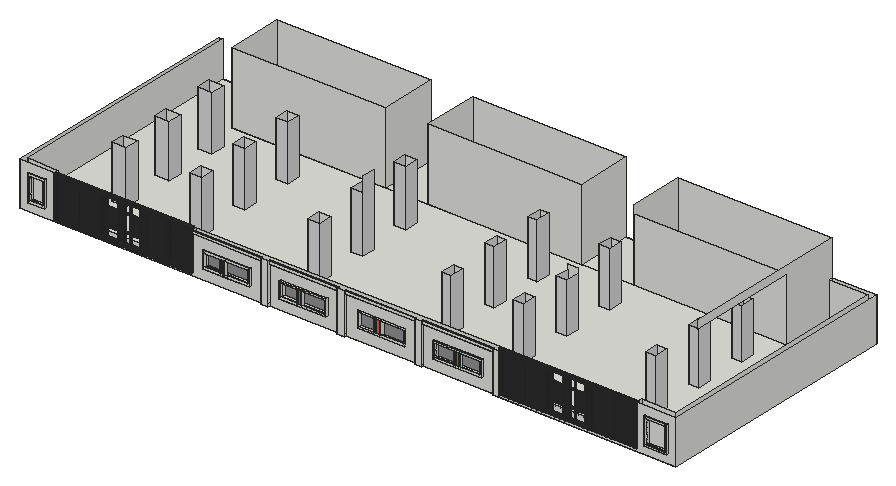
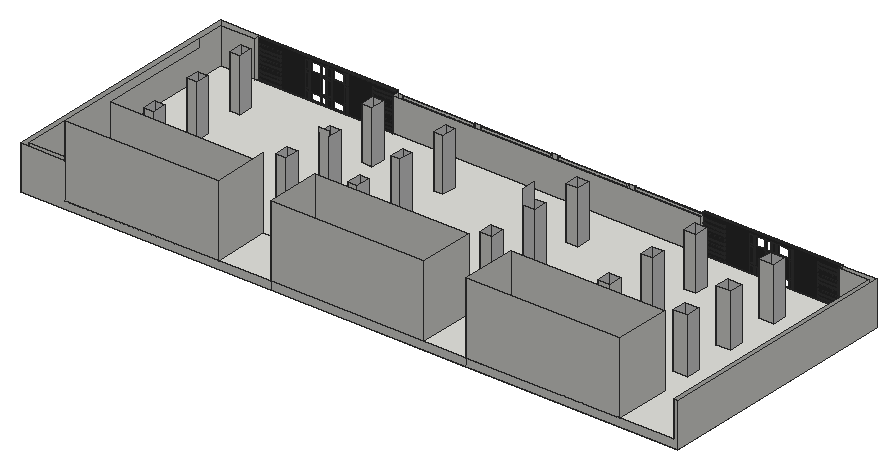
# SketchUp Ruby script. Lengths in inches.
U = 1.inch
M = Sketchup.active_model
def pt(a) = Geom::Point3d.new(a.map { |v| v * U })
def face(e, loops, mat)
  f = e.add_face(loops[0].map { |a| pt(a) })
  loops[1..].each { |l| e.add_face(l.map { |a| pt(a) }).erase! }
  f.material = f.back_material = mat if mat
  f
end
# faces: each face lists its corners as indices into pts; further lists are holes
def faces(e, pts, list, mat = nil) = list.each { |f| face(e, (f[0].is_a?(Array) ? f : [f]).map { |l| l.map { |i| pts[i] } }, mat) }
# xy, xz, yz: faces in a plane at the given z, y or x. An outline is a flat list of corners, or four numbers for a rectangle; further outlines are holes
def ring(l) = l.size == 4 ? [[l[0], l[1]], [l[2], l[1]], [l[2], l[3]], [l[0], l[3]]] : l.each_slice(2).to_a
def flat(e, list, mat, &to3) = list.each { |f| face(e, (f[0].is_a?(Array) ? f : [f]).map { |l| ring(l).map { |u, v| to3.(u, v) } }, mat) }
def xy(e, z, list, mat = nil) = flat(e, list, mat) { |x, y| [x, y, z] }
def xz(e, y, list, mat = nil) = flat(e, list, mat) { |x, z| [x, y, z] }
def yz(e, x, list, mat = nil) = flat(e, list, mat) { |y, z| [x, y, z] }
def lines(e, pts, list) = list.each { |a, b| e.add_line(pt(pts[a]), pt(pts[b])) }
# prism: a flat outline (further loops are holes) pulled along v
def prism(e, loops, v, mat = nil)
  f = face(e, loops, mat); d = Geom::Vector3d.new(v.map { |x| x * U })
  f.pushpull(f.normal.samedirection?(d) ? d.length : -d.length)
end
def box(e, o, s, mat = nil) = prism(e, [[o, [o[0] + s[0], o[1], o[2]], [o[0] + s[0], o[1] + s[1], o[2]], [o[0], o[1] + s[1], o[2]]]], [0, 0, s[2]], mat)
def at(x, y, z, deg = 0) = Geom::Transformation.translation(pt([x, y, z])) * Geom::Transformation.rotation(ORIGIN, Z_AXIS, deg.degrees)
def axes(o, x, y, z) = Geom::Transformation.new([*x, 0, *y, 0, *z, 0, *pt(o).to_a, 1])
def part(name) = M.definitions.add(name)
# library, detail: a bought-in or finely detailed component or shape, given as its bounding box
def library(name, o, s) = part(name).tap { |d| box(d.entities, o, s) }
def detail(e, o, s) = box(e.add_group.entities, o, s)
def put(e, d, t, mat = nil) = e.add_instance(d, t).tap { |i| i.material = mat if mat }
def group(e, t, mat = nil) = e.add_group.tap { |g| g.transformation = t; g.material = mat if mat }.entities
root = M.entities
M.materials.add("Generic").color = [145, 145, 145]
M.materials.add("Generic\#2").color = [229, 87, 87]
M.materials.add("Generic\#3").color = [216, 216, 216]
M.materials.add("[Color M08]").color = [45, 45, 45]
c1 = part("Group\#13")
xy(c1.entities,0,[[0,0,323.37,7]],"[Color M08]")
xy(c1.entities,5.37,[[5.37,0,53,7],[58.37,0,106,4],[111.37,0,159,0,159,7,150.06,7,150.06,4,148.06,4,148.06,7,121.81,7,121.81,4,119.81,4,119.81,7,111.37,7],[164.37,0,212,0,212,7,201.24,7,201.24,4,199.24,4,199.24,7,176.81,7,176.81,4,174.81,4,174.81,7,164.37,7],[217.37,0,265,4],
  [270.37,0,318,4]],"[Color M08]")
xy(c1.entities,8.44,[[5.37,4,53,7]])
xy(c1.entities,8.57,[[270.37,4,318,7]],"[Color M08]")
xy(c1.entities,12.19,[[270.37,4,318,7]],"[Color M08]")
xy(c1.entities,13.07,[[5.37,4,53,7]],"[Color M08]")
xy(c1.entities,16.32,[[5.37,4,53,7]],"[Color M08]")
xy(c1.entities,17.82,[[270.37,4,318,7]],"[Color M08]")
xy(c1.entities,20.94,[[5.37,4,53,7]],"[Color M08]")
xy(c1.entities,21.44,[[270.37,4,318,7]],"[Color M08]")
xy(c1.entities,24.19,[[5.37,4,53,7]],"[Color M08]")
xy(c1.entities,26.69,[[111.37,4,119.81,7],[121.81,4,148.06,7],[150.06,4,159,7],[164.37,4,174.81,7],[176.81,4,199.24,7],
  [201.24,4,212,7]],"[Color M08]")
xy(c1.entities,27.07,[[270.37,4,318,7]],"[Color M08]")
xy(c1.entities,28.82,[[5.37,4,53,7]],"[Color M08]")
xy(c1.entities,29.69,[[111.37,4,119.81,7],[150.06,4,159,7],[164.37,4,174.81,7],[201.24,4,212,7]],"[Color M08]")
xy(c1.entities,30.69,[[270.37,4,318,7]],"[Color M08]")
xy(c1.entities,32.07,[[5.37,4,53,7]],"[Color M08]")
xy(c1.entities,36.32,[[270.37,4,318,7]],"[Color M08]")
xy(c1.entities,36.69,[[5.37,4,53,7]],"[Color M08]")
xy(c1.entities,39.94,[[5.37,4,53,7],[270.37,4,318,7]],"[Color M08]")
xy(c1.entities,44.57,[[5.37,4,53,7]],"[Color M08]")
xy(c1.entities,45.57,[[270.37,4,318,7]],"[Color M08]")
xy(c1.entities,47.82,[[5.37,4,53,7]],"[Color M08]")
xy(c1.entities,49.19,[[270.37,4,318,7]],"[Color M08]")
xy(c1.entities,52.44,[[5.37,4,53,7]],"[Color M08]")
xy(c1.entities,54.82,[[270.37,4,318,7]],"[Color M08]")
xy(c1.entities,55.69,[[5.37,4,53,7]],"[Color M08]")
xy(c1.entities,58.44,[[270.37,4,318,7]],"[Color M08]")
xy(c1.entities,60.32,[[5.37,4,53,7]],"[Color M08]")
xy(c1.entities,63.57,[[5.37,4,53,7]],"[Color M08]")
xy(c1.entities,64.07,[[270.37,4,318,7]],"[Color M08]")
xy(c1.entities,66.38,[[111.37,4,119.81,7],[150.06,4,159,7],[164.37,4,174.81,7],[201.24,4,212,7]],"[Color M08]")
xy(c1.entities,67.69,[[270.37,4,318,7]],"[Color M08]")
xy(c1.entities,68.19,[[5.37,4,53,7]],"[Color M08]")
xy(c1.entities,69.38,[[111.37,4,119.81,7],[121.81,4,148.06,7],[150.06,4,159,7],[164.37,4,174.81,7],[176.81,4,199.24,7],
  [201.24,4,212,7]],"[Color M08]")
xy(c1.entities,71.44,[[5.37,4,53,7]],"[Color M08]")
xy(c1.entities,73.32,[[270.37,4,318,7]],"[Color M08]")
xy(c1.entities,76.07,[[5.37,4,53,7]],"[Color M08]")
xy(c1.entities,76.94,[[270.37,4,318,7]],"[Color M08]")
xy(c1.entities,79.32,[[5.37,4,53,7]],"[Color M08]")
xy(c1.entities,82.57,[[270.37,4,318,7]],"[Color M08]")
xy(c1.entities,83.94,[[5.37,4,53,7]],"[Color M08]")
xy(c1.entities,86.19,[[270.37,4,318,7]],"[Color M08]")
xy(c1.entities,87.19,[[5.37,4,53,7]],"[Color M08]")
xy(c1.entities,91.82,[[5.37,0,53,4],[58.37,0,106,4],[111.37,0,111.37,7,119.81,7,119.81,4,121.81,4,121.81,7,148.06,7,148.06,4,150.06,4,150.06,7,159,7,159,0],[164.37,0,164.37,7,174.81,7,174.81,4,176.81,4,176.81,7,199.24,7,199.24,4,201.24,4,201.24,7,212,7,212,0],[217.37,0,265,4],
  [270.37,0,318,4]],"[Color M08]")
xy(c1.entities,97.1875,[[0,0,323.37,7]],"[Color M08]")
xz(c1.entities,0,[[[0,0,323.37,0,323.37,97.1875,0,97.1875,0,5.37,5.37,5.37,5.37,91.82,53,91.82,53,5.37,58.37,5.37,58.37,91.82,106,91.82,106,5.37,111.37,5.37,111.37,91.82,212,91.82,212,5.37,0,5.37],[270.37,5.37,318,91.82],[217.37,5.37,265,91.82]],[159,5.37,164.37,91.82]],"[Color M08]")
xz(c1.entities,4,[[5.37,0.57,53,5.19],[270.37,2.94,318,5.37]])
xz(c1.entities,4,[[58.37,5.37,106,91.82],[119.81,5.37,121.81,5.37,121.81,26.69,148.06,26.69,148.06,5.37,150.06,5.37,150.06,26.69,159,26.69,159,29.69,150.06,29.69,150.06,66.38,159,66.38,159,69.38,150.06,69.38,150.06,91.82,148.06,91.82,148.06,69.38,121.81,69.38,121.81,91.82,119.81,91.82,119.81,69.38,111.37,69.38,111.37,66.38,119.81,66.38,119.81,29.69,121.81,29.69,121.81,66.38,148.06,66.38,148.06,29.69,111.37,29.69,111.37,26.69,119.81,26.69],[[174.81,5.37,176.81,5.37,176.81,26.69,199.24,26.69,199.24,5.37,201.24,5.37,201.24,26.69,212,26.69,212,29.69,201.24,29.69,201.24,66.38,212,66.38,212,69.38,201.24,69.38,201.24,91.82,199.24,91.82,199.24,69.38,176.81,69.38,176.81,91.82,174.81,91.82,174.81,69.38,164.37,69.38,164.37,66.38,174.81,66.38,174.81,29.69,164.37,29.69,164.37,26.69,174.81,26.69],[176.81,29.69,199.24,66.38]],[217.37,5.37,265,91.82],[270.37,5.37,318,8.57],
  [5.37,8.44,53,13.07],[270.37,12.19,318,17.82],[5.37,16.32,53,20.94],[270.37,21.44,318,27.07],[5.37,24.19,53,28.82],
  [121.81,29.69,148.06,66.38],[176.81,29.69,199.24,66.38],[270.37,30.69,318,36.32],[5.37,32.07,53,36.69],[5.37,39.94,53,44.57],
  [270.37,39.94,318,45.57],[5.37,47.82,53,52.44],[270.37,49.19,318,54.82],[5.37,55.69,53,60.32],[270.37,58.44,318,64.07],
  [5.37,63.57,53,68.19],[270.37,67.69,318,73.32],[5.37,71.44,53,76.07],[270.37,76.94,318,82.57],[5.37,79.32,53,83.94],
  [270.37,86.19,318,91.82],[5.37,87.19,53,91.82]],"[Color M08]")
xz(c1.entities,7,[[[0,0,323.37,97.1875],[121.81,69.38,148.06,91.82],[121.81,5.37,148.06,26.69],[176.81,69.38,199.24,91.82],[176.81,5.37,199.24,26.69],[201.24,29.69,212,66.38],[164.37,29.69,174.81,66.38],[150.06,29.69,159,66.38],[111.37,29.69,119.81,66.38],[201.24,69.38,212,91.82],[164.37,69.38,174.81,91.82],[201.24,5.37,212,26.69],[164.37,5.37,174.81,26.69],[150.06,69.38,159,91.82],[150.06,5.37,159,26.69],[111.37,69.38,119.81,91.82],[111.37,5.37,119.81,26.69],[270.37,82.57,318,86.19],[270.37,73.32,318,76.94],[270.37,64.07,318,67.69],[270.37,54.82,318,58.44],[270.37,45.57,318,49.19],[270.37,36.32,318,39.94],[270.37,27.07,318,30.69],[270.37,17.82,318,21.44],[270.37,8.57,318,12.19],[5.37,83.94,53,87.19],[5.37,76.07,53,79.32],[5.37,68.19,53,71.44],[5.37,60.32,53,63.57],[5.37,52.44,53,55.69],[5.37,44.57,53,47.82],[5.37,36.69,53,39.94],[5.37,28.82,53,32.07],[5.37,20.94,53,24.19],[5.37,13.07,53,16.32],[5.37,5.37,53,8.44]]],"[Color M08]")
yz(c1.entities,0,[[0,0,7,97.1875]],"[Color M08]")
yz(c1.entities,5.37,[[0,5.37,7,5.37,7,8.44,4,8.44,4,13.07,7,13.07,7,16.32,4,16.32,4,20.94,7,20.94,7,24.19,4,24.19,4,28.82,7,28.82,7,32.07,4,32.07,4,36.69,7,36.69,7,39.94,4,39.94,4,44.57,7,44.57,7,47.82,4,47.82,4,52.44,7,52.44,7,55.69,4,55.69,4,60.32,7,60.32,7,63.57,4,63.57,4,68.19,7,68.19,7,71.44,4,71.44,4,76.07,7,76.07,7,79.32,4,79.32,4,83.94,7,83.94,7,87.19,4,87.19,4,91.82,0,91.82]],"[Color M08]")
yz(c1.entities,53,[[0,5.37,0,91.82,4,91.82,4,87.19,7,87.19,7,83.94,4,83.94,4,79.32,7,79.32,7,76.07,4,76.07,4,71.44,7,71.44,7,68.19,4,68.19,4,63.57,7,63.57,7,60.32,4,60.32,4,55.69,7,55.69,7,52.44,4,52.44,4,47.82,7,47.82,7,44.57,4,44.57,4,39.94,7,39.94,7,36.69,4,36.69,4,32.07,7,32.07,7,28.82,4,28.82,4,24.19,7,24.19,7,20.94,4,20.94,4,16.32,7,16.32,7,13.07,4,13.07,4,8.44,7,8.44,7,5.37]],"[Color M08]")
yz(c1.entities,58.37,[[0,5.37,4,91.82]],"[Color M08]")
yz(c1.entities,106,[[0,5.37,4,91.82]],"[Color M08]")
yz(c1.entities,111.37,[[0,5.37,7,5.37,7,26.69,4,26.69,4,29.69,7,29.69,7,66.38,4,66.38,4,69.38,7,69.38,7,91.82,0,91.82]],"[Color M08]")
yz(c1.entities,119.81,[[4,5.37,7,26.69],[4,29.69,7,66.38],[4,69.38,7,91.82]],"[Color M08]")
yz(c1.entities,121.81,[[4,5.37,7,26.69],[4,69.38,7,91.82]],"[Color M08]")
yz(c1.entities,148.06,[[4,5.37,7,26.69],[4,69.38,7,91.82]],"[Color M08]")
yz(c1.entities,150.06,[[4,5.37,7,26.69],[4,29.69,7,66.38],[4,69.38,7,91.82]],"[Color M08]")
yz(c1.entities,159,[[0,5.37,0,91.82,7,91.82,7,69.38,4,69.38,4,66.38,7,66.38,7,29.69,4,29.69,4,26.69,7,26.69,7,5.37]],"[Color M08]")
yz(c1.entities,164.37,[[0,5.37,7,5.37,7,26.69,4,26.69,4,29.69,7,29.69,7,66.38,4,66.38,4,69.38,7,69.38,7,91.82,0,91.82]],"[Color M08]")
yz(c1.entities,174.81,[[4,5.37,7,26.69],[4,29.69,7,66.38],[4,69.38,7,91.82]],"[Color M08]")
yz(c1.entities,176.81,[[4,5.37,7,26.69],[4,69.38,7,91.82]],"[Color M08]")
yz(c1.entities,199.24,[[4,5.37,7,26.69],[4,69.38,7,91.82]],"[Color M08]")
yz(c1.entities,201.24,[[4,5.37,7,26.69],[4,29.69,7,66.38],[4,69.38,7,91.82]],"[Color M08]")
yz(c1.entities,212,[[0,5.37,0,91.82,7,91.82,7,69.38,4,69.38,4,66.38,7,66.38,7,29.69,4,29.69,4,26.69,7,26.69,7,5.37]],"[Color M08]")
yz(c1.entities,217.37,[[0,5.37,4,91.82]],"[Color M08]")
yz(c1.entities,265,[[0,5.37,4,91.82]],"[Color M08]")
yz(c1.entities,270.37,[[0,5.37,4,5.37,4,8.57,7,8.57,7,12.19,4,12.19,4,17.82,7,17.82,7,21.44,4,21.44,4,27.07,7,27.07,7,30.69,4,30.69,4,36.32,7,36.32,7,39.94,4,39.94,4,45.57,7,45.57,7,49.19,4,49.19,4,54.82,7,54.82,7,58.44,4,58.44,4,64.07,7,64.07,7,67.69,4,67.69,4,73.32,7,73.32,7,76.94,4,76.94,4,82.57,7,82.57,7,86.19,4,86.19,4,91.82,0,91.82]],"[Color M08]")
yz(c1.entities,318,[[0,5.37,0,91.82,4,91.82,4,86.19,7,86.19,7,82.57,4,82.57,4,76.94,7,76.94,7,73.32,4,73.32,4,67.69,7,67.69,7,64.07,4,64.07,4,58.44,7,58.44,7,54.82,4,54.82,4,49.19,7,49.19,7,45.57,4,45.57,4,39.94,7,39.94,7,36.32,4,36.32,4,30.69,7,30.69,7,27.07,4,27.07,4,21.44,7,21.44,7,17.82,4,17.82,4,12.19,7,12.19,7,8.57,4,8.57,4,5.37]],"[Color M08]")
yz(c1.entities,323.37,[[0,0,7,97.1875]],"[Color M08]")
xy(root,-18.4375,[[566.41,4.0625,566.41,8.375,495.5,8.375,495.5,590.625,954.11,590.625,954.11,8.375,943.95,8.375,943.95,4.0625,927.64,4.0625,927.64,8.375,763.9,8.375,763.9,4.0625,746.02,4.0625,746.02,8.375,583.85,8.375,583.85,4.0625],[1109.75,4.0625,1109.75,8.375,954.11,8.375,954.11,590.625,1540.27,590.625,1540.27,4.0625],[0,8.375,495.5,590.625]])
xy(root,-13.1875,[[1124,4.0625,1447.36,19.0625],[80.43,8.375,403.8,19.0625]])
xy(root,0,[[[8.1875,19.0625,1528.71,19.0625,1528.71,580.6875,1435.83,580.6875,1435.83,459.8125,135.5,459.8125,135.5,590.625,8.1875,590.625],[135.5,359.61,168.88,392.11],[135.5,233.58,168.88,266.08],[135.5,107.54,168.88,140.04],[594.11,359.61,622.68,392.11],[594.11,233.58,622.68,266.08],[594.11,107.54,622.68,140.04],[317.97,359.61,346.15,392.11],[317.97,233.58,346.15,266.08],[317.97,107.54,346.15,140.04],[1075.83,359.61,1100.54,392.11],[1075.83,233.58,1100.54,266.08],[1075.83,107.54,1100.54,140.04],[1385.5,359.61,1409.07,392.11],[1385.5,233.58,1409.07,266.08],[1385.5,107.54,1409.07,140.04],[909.52,359.61,930.58,392.11],[909.52,233.58,930.58,266.08],[909.52,107.54,930.58,140.04]],[135.5,107.54,168.88,140.04],[594.11,107.54,622.68,140.04],[909.52,107.54,930.58,140.04],[1075.83,107.54,1100.54,140.04],
  [1385.5,107.54,1409.07,140.04],[594.11,233.58,622.68,266.08],[909.52,233.58,930.58,266.08],[1075.83,233.58,1100.54,266.08],[1385.5,233.58,1409.07,266.08],
  [594.11,359.61,622.68,392.11],[909.52,359.61,930.58,392.11],[1075.83,359.61,1100.54,392.11],[1385.5,359.61,1409.07,392.11],[135.5,459.8125,495.5,590.625],
  [495.5,459.8125,594.11,590.625],[594.11,459.8125,954.11,590.625],[954.11,459.8125,1075.83,590.625],[1075.83,459.8125,1435.83,590.625]])
xy(root,1.18,[[1466.98,0,1520.66,4.0625]])
xy(root,2.02,[[20.45,4.3125,59.98,8.375]])
xy(root,4.8,[[1470.6,0,1517.04,4.0625],[1470.6,4.0625,1517.04,10.25]])
xy(root,6.4,[[24.84,4.3125,55.59,8.375],[24.84,8.375,55.59,14.5625]])
xy(root,7.54,[[429.78,4.3125,495.5,8.375],[495.5,4.3125,540.43,8.375],[609.83,4.3125,720.04,8.375],[969.93,4.3125,1083.77,8.375]])
xy(root,11.55,[[433.78,4.3125,469.65,8.375],[469.65,4.3125,473.97,8.375],[473.97,4.3125,478.71,8.375],[478.71,4.3125,483.02,8.375],[483.02,4.3125,536.43,8.375],
  [613.83,4.3125,650.42,8.375],[650.42,4.3125,654.36,8.375],[654.36,4.3125,659.51,8.375],[659.51,4.3125,663.45,8.375],[663.45,4.3125,716.04,8.375],
  [973.93,4.3125,1020.07,8.375],[1020.07,4.3125,1023.76,8.375],[1023.76,4.3125,1030.95,8.375],[1030.95,4.3125,1034.64,8.375],[1034.64,4.3125,1079.76,8.375],
  [433.78,8.375,536.43,14.5625],[613.83,8.375,716.04,14.5625],[793.88,8.375,829.46,14.5625],[829.46,8.375,833.9,14.5625],[833.9,8.375,841.35,14.5625],
  [841.35,8.375,845.78,14.5625],[845.78,8.375,897.65,14.5625],[973.93,8.375,1079.76,14.5625]])
xy(root,41.52,[[433.78,4.3125,469.65,8.375],[469.65,4.3125,473.97,8.375],[473.97,4.3125,478.71,8.375],[478.71,4.3125,483.02,8.375],[483.02,4.3125,536.43,8.375],
  [613.83,4.3125,650.42,8.375],[650.42,4.3125,654.36,8.375],[654.36,4.3125,659.51,8.375],[659.51,4.3125,663.45,8.375],[663.45,4.3125,716.04,8.375],
  [973.93,4.3125,1020.07,8.375],[1020.07,4.3125,1023.76,8.375],[1023.76,4.3125,1030.95,8.375],[1030.95,4.3125,1034.64,8.375],[1034.64,4.3125,1079.76,8.375],
  [433.78,8.375,536.43,14.5625],[613.83,8.375,716.04,14.5625],[793.88,8.375,829.46,14.5625],[829.46,8.375,833.9,14.5625],[833.9,8.375,841.35,14.5625],
  [841.35,8.375,845.78,14.5625],[845.78,8.375,897.65,14.5625],[973.93,8.375,1079.76,14.5625]])
xy(root,45.52,[[429.78,4.3125,540.43,8.375],[609.83,4.3125,720.04,8.375],[969.93,4.3125,1083.77,8.375]])
xy(root,59.16,[[24.84,4.3125,55.59,8.375],[24.84,8.375,55.59,14.5625]])
xy(root,60.77,[[1470.6,0,1517.04,4.0625],[1470.6,4.0625,1517.04,10.25]])
xy(root,63.55,[[20.45,4.3125,59.98,8.375]])
xy(root,64.39,[[1466.98,0,1520.66,4.0625]])
xy(root,71.5,[[403.8,5.5,566.41,8.375],[583.85,5.5,746.02,8.375],[763.9,5.5,927.64,8.375],[943.95,5.5,1109.75,8.375]])
xz(root,0,[[[1466.98,1.18,1520.66,64.39],[1470.6,4.8,1517.04,60.77]]])
xz(root,4.0625,[[566.41,-18.4375,583.85,77.4375],[746.02,-18.4375,763.9,77.4375],[927.64,-18.4375,943.95,77.4375],[1109.75,-18.4375,1124,77.4375],[[1124,-18.4375,1540.27,-18.4375,1540.27,84,1447.36,84,1447.36,-13.1875,1124,-13.1875],[1466.98,1.18,1520.66,64.39]],
  [[1466.98,1.18,1520.66,64.39],[1470.6,4.8,1517.04,60.77]]])
xz(root,4.3125,[[[20.45,2.02,59.98,63.55],[24.84,6.4,55.59,59.16]],[[429.78,7.54,540.43,45.52],[433.78,11.55,536.43,41.52]],[[609.83,7.54,720.04,45.52],[613.83,11.55,716.04,41.52]],[[969.93,7.54,1083.77,45.52],[973.93,11.55,1079.76,41.52]],[469.65,11.55,473.97,41.52],
  [478.71,11.55,483.02,41.52],[650.42,11.55,654.36,41.52],[659.51,11.55,663.45,41.52],[1020.07,11.55,1023.76,41.52],[1030.95,11.55,1034.64,41.52]])
xz(root,4.3125,[[473.97,11.55,478.71,41.52],[654.36,11.55,659.51,41.52],[1023.76,11.55,1030.95,41.52]],"Generic\#2")
xz(root,5.5,[[403.8,71.5,566.41,77.4375],[583.85,71.5,746.02,77.4375],[763.9,71.5,927.64,77.4375],[943.95,71.5,1109.75,77.4375]])
xz(root,8.375,[[[0,-18.4375,566.41,-18.4375,566.41,71.5,403.8,71.5,403.8,-13.1875,80.43,-13.1875,80.43,84,0,84],[429.78,7.54,540.43,45.52],[20.45,2.02,59.98,63.55]],[[583.85,-18.4375,746.02,71.5],[609.83,7.54,720.04,45.52]],[[763.9,-18.4375,927.64,71.5],[789.88,7.54,901.65,45.52]],[[943.95,-18.4375,1109.75,71.5],[969.93,7.54,1083.77,45.52]],[[20.45,2.02,59.98,63.55],[24.84,6.4,55.59,59.16]],
  [[429.78,7.54,540.43,45.52],[433.78,11.55,536.43,41.52]],[[609.83,7.54,720.04,45.52],[613.83,11.55,716.04,41.52]],[[789.88,7.54,901.65,45.52],[793.88,11.55,897.65,41.52]],[[969.93,7.54,1083.77,45.52],[973.93,11.55,1079.76,41.52]],[469.65,11.55,473.97,41.52],
  [473.97,11.55,478.71,41.52],[478.71,11.55,483.02,41.52],[650.42,11.55,654.36,41.52],[654.36,11.55,659.51,41.52],[659.51,11.55,663.45,41.52],
  [829.46,11.55,833.9,41.52],[841.35,11.55,845.78,41.52],[1020.07,11.55,1023.76,41.52],[1023.76,11.55,1030.95,41.52],[1030.95,11.55,1034.64,41.52],
  [403.8,71.5,566.41,77.4375],[583.85,71.5,746.02,77.4375],[763.9,71.5,927.64,77.4375],[943.95,71.5,1109.75,77.4375]])
xz(root,8.375,[[833.9,11.55,841.35,41.52]],"Generic\#2")
xz(root,10.25,[[1470.6,4.8,1517.04,60.77]])
xz(root,14.5625,[[24.84,6.4,55.59,59.16],[829.46,11.55,833.9,41.52],[833.9,11.55,841.35,41.52],[841.35,11.55,845.78,41.52]])
xz(root,14.5625,[[433.78,11.55,536.43,41.52],[613.83,11.55,716.04,41.52],[793.88,11.55,829.46,41.52],[845.78,11.55,897.65,41.52],[973.93,11.55,1079.76,41.52]],"Generic")
xz(root,19.0625,[[80.43,-13.1875,403.8,0],[1124,-13.1875,1447.36,0],[8.1875,0,80.43,84],[403.8,0,1124,77.4375],[1447.36,0,1528.71,84]])
xz(root,107.54,[[135.5,0,168.88,123.46],[317.97,0,346.15,123.46],[594.11,0,622.68,123.46],[909.52,0,930.58,123.46],[1075.83,0,1100.54,123.46],
  [1385.5,0,1409.07,123.46]],"Generic\#3")
xz(root,140.04,[[135.5,0,168.88,123.46],[317.97,0,346.15,123.46],[594.11,0,622.68,123.46],[909.52,0,930.58,123.46],[1075.83,0,1100.54,123.46],
  [1385.5,0,1409.07,123.46]])
xz(root,233.58,[[135.5,0,168.88,123.46],[317.97,0,346.15,128.98],[594.11,0,622.68,133.04],[909.52,0,930.58,128.98],[1075.83,0,1100.54,117.37],
  [1385.5,0,1409.07,123.46]],"Generic\#3")
xz(root,266.08,[[135.5,0,168.88,123.46],[317.97,0,346.15,128.98],[909.52,0,930.58,128.98],[1075.83,0,1100.54,128.98],[1385.5,0,1409.07,123.46]])
xz(root,266.08,[[594.11,0,622.68,133.04]],"Generic\#3")
xz(root,359.61,[[135.5,0,168.88,128.98],[317.97,0,346.15,128.98],[594.11,0,622.68,132.52],[909.52,0,930.58,128.98],[1075.83,0,1100.54,128.98],
  [1385.5,0,1409.07,117.37]],"Generic\#3")
xz(root,392.11,[[135.5,0,168.88,128.98],[317.97,0,346.15,128.98],[594.11,0,622.68,132.52],[909.52,0,930.58,128.98],[1075.83,0,1100.54,128.98],
  [1385.5,0,1409.07,117.37]])
xz(root,459.8125,[[135.5,0,495.5,168],[594.11,0,954.11,168],[1075.83,0,1435.83,148.75]])
xz(root,580.6875,[[1435.83,0,1528.71,84]])
xz(root,590.625,[[0,-18.4375,0,84,8.1875,84,8.1875,0,495.5,0,495.5,-18.4375],[495.5,-18.4375,954.11,0],[954.11,-18.4375,954.11,0,1435.83,0,1435.83,84,1540.27,84,1540.27,-18.4375],[135.5,0,495.5,168],[594.11,0,954.11,168],
  [1075.83,0,1435.83,168]])
yz(root,0,[[8.375,-18.4375,590.625,84]])
yz(root,8.1875,[[19.0625,0,590.625,84]])
yz(root,20.45,[[4.3125,2.02,8.375,63.55]])
yz(root,24.84,[[4.3125,6.4,8.375,59.16],[8.375,6.4,14.5625,59.16]])
yz(root,55.59,[[4.3125,6.4,8.375,59.16],[8.375,6.4,14.5625,59.16]])
yz(root,59.98,[[4.3125,2.02,8.375,63.55]])
yz(root,80.43,[[8.375,-13.1875,19.0625,84]])
yz(root,135.5,[[459.8125,0,590.625,168]])
yz(root,135.5,[[107.54,0,140.04,123.46],[233.58,0,266.08,123.46],[359.61,0,392.11,128.98]],"Generic\#3")
yz(root,168.88,[[107.54,0,140.04,123.46],[233.58,0,266.08,123.46],[359.61,0,392.11,128.98]],"Generic\#3")
yz(root,317.97,[[359.61,0,392.11,128.98]])
yz(root,317.97,[[107.54,0,140.04,123.46],[233.58,0,266.08,128.98]],"Generic\#3")
yz(root,346.15,[[107.54,0,140.04,123.46],[233.58,0,266.08,128.98],[359.61,0,392.11,128.98]],"Generic\#3")
yz(root,403.8,[[8.375,-13.1875,19.0625,77.4375],[5.5,71.5,8.375,77.4375]])
yz(root,429.78,[[4.3125,7.54,8.375,45.52]])
yz(root,433.78,[[4.3125,11.55,8.375,41.52],[8.375,11.55,14.5625,41.52]])
yz(root,469.65,[[4.3125,11.55,8.375,41.52]])
yz(root,473.97,[[4.3125,11.55,8.375,41.52]])
yz(root,478.71,[[4.3125,11.55,8.375,41.52]])
yz(root,483.02,[[4.3125,11.55,8.375,41.52]])
yz(root,495.5,[[459.8125,0,590.625,168]])
yz(root,536.43,[[4.3125,11.55,8.375,41.52],[8.375,11.55,14.5625,41.52]])
yz(root,540.43,[[4.3125,7.54,8.375,45.52]])
yz(root,566.41,[[4.0625,-18.4375,8.375,-13.1875],[4.0625,-13.1875,4.0625,77.4375,5.5,77.4375,5.5,71.5,8.375,71.5,8.375,-13.1875],[5.5,71.5,8.375,77.4375]])
yz(root,583.85,[[4.0625,-18.4375,8.375,-13.1875],[4.0625,-13.1875,8.375,-13.1875,8.375,71.5,5.5,71.5,5.5,77.4375,4.0625,77.4375],[5.5,71.5,8.375,77.4375]])
yz(root,594.11,[[459.8125,0,590.625,168]])
yz(root,594.11,[[107.54,0,140.04,123.46],[233.58,0,266.08,133.04],[359.61,0,392.11,132.52]],"Generic\#3")
yz(root,609.83,[[4.3125,7.54,8.375,45.52]])
yz(root,613.83,[[4.3125,11.55,8.375,41.52],[8.375,11.55,14.5625,41.52]])
yz(root,622.68,[[107.54,0,140.04,123.46],[233.58,0,266.08,168],[359.61,0,392.11,132.52]],"Generic\#3")
yz(root,650.42,[[4.3125,11.55,8.375,41.52]])
yz(root,654.36,[[4.3125,11.55,8.375,41.52]])
yz(root,659.51,[[4.3125,11.55,8.375,41.52]])
yz(root,663.45,[[4.3125,11.55,8.375,41.52]])
yz(root,716.04,[[4.3125,11.55,8.375,41.52],[8.375,11.55,14.5625,41.52]])
yz(root,720.04,[[4.3125,7.54,8.375,45.52]])
yz(root,746.02,[[4.0625,-18.4375,8.375,-13.1875],[4.0625,-13.1875,4.0625,77.4375,5.5,77.4375,5.5,71.5,8.375,71.5,8.375,-13.1875],[5.5,71.5,8.375,77.4375]])
yz(root,763.9,[[4.0625,-18.4375,8.375,-13.1875],[4.0625,-13.1875,8.375,-13.1875,8.375,71.5,5.5,71.5,5.5,77.4375,4.0625,77.4375],[5.5,71.5,8.375,77.4375]])
yz(root,793.88,[[8.375,11.55,14.5625,41.52]])
yz(root,829.46,[[8.375,11.55,14.5625,41.52]])
yz(root,833.9,[[8.375,11.55,14.5625,41.52]])
yz(root,841.35,[[8.375,11.55,14.5625,41.52]])
yz(root,845.78,[[8.375,11.55,14.5625,41.52]])
yz(root,897.65,[[8.375,11.55,14.5625,41.52]])
yz(root,909.52,[[107.54,0,140.04,123.46],[233.58,0,266.08,128.98],[359.61,0,392.11,128.98]],"Generic\#3")
yz(root,927.64,[[4.0625,-18.4375,8.375,-13.1875],[4.0625,-13.1875,4.0625,77.4375,5.5,77.4375,5.5,71.5,8.375,71.5,8.375,-13.1875],[5.5,71.5,8.375,77.4375]])
yz(root,930.58,[[107.54,0,140.04,123.46],[233.58,0,266.08,128.98],[359.61,0,392.11,128.98]],"Generic\#3")
yz(root,943.95,[[4.0625,-18.4375,8.375,-13.1875],[4.0625,-13.1875,8.375,-13.1875,8.375,71.5,5.5,71.5,5.5,77.4375,4.0625,77.4375],[5.5,71.5,8.375,77.4375]])
yz(root,954.11,[[459.8125,0,590.625,168]])
yz(root,969.93,[[4.3125,7.54,8.375,45.52]])
yz(root,973.93,[[4.3125,11.55,8.375,41.52],[8.375,11.55,14.5625,41.52]])
yz(root,1020.07,[[4.3125,11.55,8.375,41.52]])
yz(root,1023.76,[[4.3125,11.55,8.375,41.52]])
yz(root,1030.95,[[4.3125,11.55,8.375,41.52]])
yz(root,1034.64,[[4.3125,11.55,8.375,41.52]])
yz(root,1075.83,[[459.8125,0,590.625,168]])
yz(root,1075.83,[[107.54,0,140.04,123.46],[233.58,0,266.08,117.37],[359.61,0,392.11,128.98]],"Generic\#3")
yz(root,1079.76,[[4.3125,11.55,8.375,41.52],[8.375,11.55,14.5625,41.52]])
yz(root,1083.77,[[4.3125,7.54,8.375,45.52]])
yz(root,1100.54,[[107.54,0,140.04,123.46],[233.58,0,266.08,117.37],[359.61,0,392.11,128.98]],"Generic\#3")
yz(root,1109.75,[[4.0625,-18.4375,8.375,-13.1875],[4.0625,-13.1875,4.0625,77.4375,5.5,77.4375,5.5,71.5,8.375,71.5,8.375,-13.1875],[5.5,71.5,8.375,77.4375]])
yz(root,1124,[[4.0625,-13.1875,19.0625,77.4375]])
yz(root,1385.5,[[107.54,0,140.04,123.46],[233.58,0,266.08,123.46],[359.61,0,392.11,117.37]],"Generic\#3")
yz(root,1409.07,[[107.54,0,140.04,123.46],[233.58,0,266.08,123.46],[359.61,0,392.11,117.37]],"Generic\#3")
yz(root,1435.83,[[459.8125,0,580.6875,0,580.6875,84,590.625,84,590.625,168,199.25,168,199.25,148.75,459.8125,148.75]])
yz(root,1447.36,[[4.0625,-13.1875,19.0625,84]])
yz(root,1466.98,[[0,1.18,4.0625,64.39]])
yz(root,1470.6,[[0,4.8,4.0625,60.77],[4.0625,4.8,10.25,60.77]])
yz(root,1517.04,[[0,4.8,4.0625,60.77],[4.0625,4.8,10.25,60.77]])
yz(root,1520.66,[[0,1.18,4.0625,64.39]])
yz(root,1528.71,[[19.0625,0,580.6875,84]])
yz(root,1540.27,[[4.0625,-18.4375,590.625,84]])
put(root,c1,at(1124,4.0625,-13.1875))
put(root,c1,at(80.43,5.5625,-13.1875))
